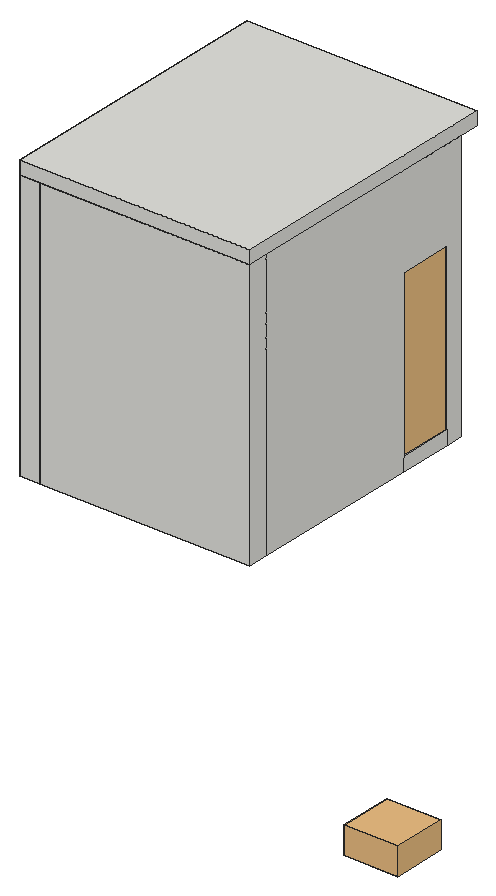
# SketchUp Ruby script. Lengths in inches.
U = 1.inch
M = Sketchup.active_model
def pt(a) = Geom::Point3d.new(a.map { |v| v * U })
def face(e, loops, mat)
  f = e.add_face(loops[0].map { |a| pt(a) })
  loops[1..].each { |l| e.add_face(l.map { |a| pt(a) }).erase! }
  f.material = f.back_material = mat if mat
  f
end
# faces: each face lists its corners as indices into pts; further lists are holes
def faces(e, pts, list, mat = nil) = list.each { |f| face(e, (f[0].is_a?(Array) ? f : [f]).map { |l| l.map { |i| pts[i] } }, mat) }
# xy, xz, yz: faces in a plane at the given z, y or x. An outline is a flat list of corners, or four numbers for a rectangle; further outlines are holes
def ring(l) = l.size == 4 ? [[l[0], l[1]], [l[2], l[1]], [l[2], l[3]], [l[0], l[3]]] : l.each_slice(2).to_a
def flat(e, list, mat, &to3) = list.each { |f| face(e, (f[0].is_a?(Array) ? f : [f]).map { |l| ring(l).map { |u, v| to3.(u, v) } }, mat) }
def xy(e, z, list, mat = nil) = flat(e, list, mat) { |x, y| [x, y, z] }
def xz(e, y, list, mat = nil) = flat(e, list, mat) { |x, z| [x, y, z] }
def yz(e, x, list, mat = nil) = flat(e, list, mat) { |y, z| [x, y, z] }
def lines(e, pts, list) = list.each { |a, b| e.add_line(pt(pts[a]), pt(pts[b])) }
# prism: a flat outline (further loops are holes) pulled along v
def prism(e, loops, v, mat = nil)
  f = face(e, loops, mat); d = Geom::Vector3d.new(v.map { |x| x * U })
  f.pushpull(f.normal.samedirection?(d) ? d.length : -d.length)
end
def box(e, o, s, mat = nil) = prism(e, [[o, [o[0] + s[0], o[1], o[2]], [o[0] + s[0], o[1] + s[1], o[2]], [o[0], o[1] + s[1], o[2]]]], [0, 0, s[2]], mat)
def at(x, y, z, deg = 0) = Geom::Transformation.translation(pt([x, y, z])) * Geom::Transformation.rotation(ORIGIN, Z_AXIS, deg.degrees)
def axes(o, x, y, z) = Geom::Transformation.new([*x, 0, *y, 0, *z, 0, *pt(o).to_a, 1])
def part(name) = M.definitions.add(name)
# library, detail: a bought-in or finely detailed component or shape, given as its bounding box
def library(name, o, s) = part(name).tap { |d| box(d.entities, o, s) }
def detail(e, o, s) = box(e.add_group.entities, o, s)
def put(e, d, t, mat = nil) = e.add_instance(d, t).tap { |i| i.material = mat if mat }
def group(e, t, mat = nil) = e.add_group.tap { |g| g.transformation = t; g.material = mat if mat }.entities
root = M.entities
M.materials.add("ATBTOALHA").color = [214, 222, 215]
M.materials.add("Aluminum_Bumpy_5cm\#2").color = [83, 85, 85]
M.materials.add("Material \#2145965240").color = [200, 201, 192]
M.materials.add("Material \#2145965245").color = [91, 110, 63]
M.materials.add("Material \#33").color = [95, 70, 46]
M.materials.add("Material \#34").color = [97, 116, 28]
M.materials.add("R842VGX RIFLESSO CARPET 200X300 SMOKE").color = [156, 152, 152]
M.materials.add("TEXTURE").color = [202, 201, 217]
M.materials.add("TEXTURE\#1").color = [208, 182, 215]
M.materials.add("TEXTURE\#2").color = [208, 164, 194]
M.materials.add("TILE").color = [214, 172, 168]
M.materials.add("Wood_232").color = [187, 187, 187]
M.materials.add("[Color M07]").color = [58, 58, 58]
M.materials.add("[Mirror 01]").color = [185, 185, 185]
M.materials.add("[Stone Vein Gray]").color = [166, 165, 165]
M.materials.add("glass").color = [129, 129, 129]
M.materials["glass"].alpha = 0.1
M.materials.add("mirror\#1").color = [129, 129, 129]
M.materials.add("staklo kabina1").color = [198, 204, 204]
M.materials["staklo kabina1"].alpha = 0.1
c1 = library("Cabinet pull",[-0.17,-0.54,-0.33],[4.53,0.54,0.66])
c2 = library("K-16141 Revival® toilet tissue holder",[-4.0625,-2.67,-4.49],[8.125,5.34,8.98])
c3 = part("Group\#48")
xy(c3.entities,0,[[0,0,0.39,22.64]])
xy(c3.entities,78.54,[[0,0,0.39,22.64]])
xz(c3.entities,0,[[0,0,0.39,78.54]])
xz(c3.entities,22.64,[[0,0,0.39,78.54]])
yz(c3.entities,0,[[0,0,22.64,78.54]])
yz(c3.entities,0.39,[[0,0,22.64,78.54]],"glass")
c4 = part("Shower screen")
put(c4.entities,c3,axes([1.18,7.5625,0.2],[1,0,0],[0,0.83439,0],[0,0,1]),"staklo kabina1")
g1 = group(c4.entities,at(1.77,49.04,22.15),"Aluminum_Bumpy_5cm\#2")
prism(g1,[[[-0.1875,2.58,48.72],[-0.1875,2.58,47.74],[-0.1875,1.44,47.74],[-0.1875,1.44,46.26],[-0.1875,2.58,46.26],[-0.1875,2.58,45.28],[-0.1875,0,45.28],[-0.1875,0,48.72]]],[0.1875,0,0],"Aluminum_Bumpy_5cm\#2")
prism(g1,[[[-0.6,2.58,45.28],[-0.6,2.58,46.26],[-0.6,1.44,46.26],[-0.6,1.44,47.74],[-0.6,2.58,47.74],[-0.6,2.58,48.72],[-0.6,0,48.72],[-0.6,0,45.28]]],[-0.1875,0,0],"Aluminum_Bumpy_5cm\#2")
prism(g1,[[[0,2.58,-14.15],[0,2.58,-13.17],[0,1.44,-13.17],[0,1.44,-11.69],[0,2.58,-11.69],[0,2.58,-10.71],[0,0,-10.71],[0,0,-14.15]]],[-0.1875,0,0],"Aluminum_Bumpy_5cm\#2")
prism(g1,[[[-0.6,2.58,-14.15],[-0.6,2.58,-13.17],[-0.6,1.44,-13.17],[-0.6,1.44,-11.69],[-0.6,2.58,-11.69],[-0.6,2.58,-10.71],[-0.6,0,-10.71],[-0.6,0,-14.15]]],[-0.1875,0,0],"Aluminum_Bumpy_5cm\#2")
xy(g1,-22.15,[[-0.79,2.64,-0.79,5.16,-0.6,5.16,-0.6,2.86,-0.1875,2.86,-0.1875,5.16,0,5.16,0,2.64]],"Aluminum_Bumpy_5cm\#2")
xy(g1,-13.12,[[-0.75,1.49,-0.04,2.64]],"Aluminum_Bumpy_5cm\#2")
xy(g1,-11.74,[[-0.75,1.49,-0.04,2.64]],"Aluminum_Bumpy_5cm\#2")
xy(g1,46.31,[[-0.75,1.49,-0.04,2.64]],"Aluminum_Bumpy_5cm\#2")
xy(g1,47.6875,[[-0.75,1.49,-0.04,2.64]],"Aluminum_Bumpy_5cm\#2")
xy(g1,56.59,[[-0.79,2.64,0,2.64,0,5.16,-0.1875,5.16,-0.1875,2.86,-0.6,2.86,-0.6,5.16,-0.79,5.16]],"Aluminum_Bumpy_5cm\#2")
xz(g1,1.49,[[-0.75,-13.12,-0.04,-11.74],[-0.75,46.31,-0.04,47.6875]],"Aluminum_Bumpy_5cm\#2")
xz(g1,2.64,[[-0.79,-22.15,0,-22.15,0,-13.12,-0.75,-13.12,-0.75,-11.74,0,-11.74,0,-10.71,-0.79,-10.71],[-0.75,-13.12,-0.04,-11.74],[-0.04,-13.12,0,-11.74],[-0.79,-10.71,0,-10.71,0,46.31,-0.75,46.31,-0.75,47.6875,0,47.6875,0,56.59,-0.79,56.59],[-0.75,46.31,-0.04,47.6875],
  [-0.04,46.31,0,47.6875]],"Aluminum_Bumpy_5cm\#2")
xz(g1,2.86,[[-0.6,-22.15,-0.1875,-10.71],[-0.6,-10.71,-0.1875,56.59]],"Aluminum_Bumpy_5cm\#2")
xz(g1,5.16,[[-0.79,-22.15,-0.6,-10.71],[-0.1875,-22.15,0,-10.71],[-0.79,-10.71,-0.6,56.59],[-0.1875,-10.71,0,56.59]],"Aluminum_Bumpy_5cm\#2")
yz(g1,-0.79,[[2.64,-22.15,5.16,56.59]],"Aluminum_Bumpy_5cm\#2")
yz(g1,-0.75,[[1.49,-13.12,2.64,-11.74],[1.49,46.31,2.64,47.6875]],"Aluminum_Bumpy_5cm\#2")
yz(g1,-0.6,[[2.86,-22.15,5.16,-10.71],[2.86,-10.71,5.16,56.59]],"Aluminum_Bumpy_5cm\#2")
yz(g1,-0.1875,[[2.86,-22.15,5.16,-10.71],[2.86,-10.71,5.16,56.59]],"Aluminum_Bumpy_5cm\#2")
yz(g1,-0.04,[[1.49,-13.12,2.64,-11.74],[1.49,46.31,2.64,47.6875]],"Aluminum_Bumpy_5cm\#2")
yz(g1,0,[[2.64,-22.15,5.16,-10.71],[2.64,-10.71,5.16,56.59]],"Aluminum_Bumpy_5cm\#2")
put(c4.entities,c3,axes([1.18,32.8,0.2],[1,0,0],[0,0.83439,0],[0,0,1]),"staklo kabina1")
c5 = library("Soap Dispenser 22-65",[-1.36,-1.375,0],[2.72,2.74,6.26])
c6 = library("Soap Dispenser 22-61",[-1.33,-1.57,0],[2.66,2.9,5.94])
c7 = library("Bath Accessories 003",[-1.27,-0.78,0],[2.49,1.57,5.35])
c8 = part("taoru")
prism(c8.entities,[[[8.78,1.24,0],[8.78,9.36,0],[8.78,9.36,1.08],[8.78,9.87,1.08],[8.78,9.87,2.17],[8.78,7.84,2.48],[8.78,1.24,2.48],[8.78,0.36,2.12],[8.78,0,1.24],[8.78,0.36,0.36]]],[-8.78,0,0],"ATBTOALHA")
p = [[0,9.36,1.08],[0,1.09,1.08],[8.78,9.36,1.08],[8.78,1.16,1.08]]
lines(c8.entities,p,[[0,1],[2,3]])
c9 = library("skp31A6",[-6.04,-1.48,32.125],[7.16,7.43,5.2])
c10 = library("skp31A6\#1",[-6.04,-1.48,32.125],[7.16,7.43,5.2])
c11 = library("PLANT-201_Defintion",[-475.32,-472.83,-28.125],[950.75,945.66,1000])
c12 = part("Group6\#1")
put(c12.entities,c11,axes([-44342.57,-2801.69,26416.98],[1.62038,0,0],[0,1.62038,0],[0,0,1.62038]),"Material \#2145965240")
c13 = library("PLANT-203_Defintion2",[-533.5,-493.98,-28.55],[984.83,1000,699.26])
c14 = library("PLANT-203_Defintion",[-526.625,-500.29,-11.57],[977.76,1000,668.71])
c15 = part("Group8\#3")
put(c15.entities,c13,axes([-44281.1875,-2905.46,27781.71],[0.88641,-1.61253,0],[1.61253,0.88641,0],[0,0,1.8685]),"Material \#34")
put(c15.entities,c14,axes([-44281.1875,-2905.46,27781.71],[0.9729,-1.76986,0],[1.76986,0.9729,0],[0,0,2.0508]),"Material \#2145965245")
c16 = part("Group7\#1")
put(c16.entities,c15,at(0,0,0))
c17 = library("PLANT-202_Defintion",[-500,-500,-15.45],[999.99,1000,259.15])
c18 = part("Group9\#1")
put(c18.entities,c17,axes([-44334.28,-2800.6875,27750.31],[0,1.46952,0],[-1.46952,0,0],[0,0,1.13496]),"Material \#33")
c19 = part("Group5\#1")
put(c19.entities,c12,at(0,0,0))
put(c19.entities,c16,at(0,0,0))
put(c19.entities,c18,at(0,0,0))
c20 = part("PLANTING")
g2 = group(c20.entities,at(4454.16,289.51,-2634.93))
put(g2,c19,axes([0,0,0],[0.1,0,0],[0,0.1,0],[0,0,0.1]))
c21 = part("DDR842RVS01100X")
xy(c21.entities,0,[[-70.87,0,47.24,78.74]])
xy(c21.entities,0.39,[[-70.87,0,47.24,78.74]],"R842VGX RIFLESSO CARPET 200X300 SMOKE")
xz(c21.entities,0,[[-70.87,0,47.24,0.39]])
xz(c21.entities,78.74,[[-70.87,0,47.24,0.39]])
yz(c21.entities,-70.87,[[0,0,78.74,0.39]])
yz(c21.entities,47.24,[[0,0,78.74,0.39]])
c22 = library("OralB_Pro6000_Toothbrush",[-0.05,-0.01,-0.01],[13.51,3.44,10.23])
c23 = library("Dome Light",[-12,-12,0],[24,24,12])
c24 = library("Group\#6",[0,0,-9.3125],[12,18,14.04])
c25 = library("Group\#15",[0,0,0],[24.35,24.35,4.73])
c26 = library("Group\#73",[0.12,0.01,0],[2.52,3.27,6.75])
c27 = library("组\#30",[-0.73,0,0],[12.16,12.33,14.02])
c28 = library("Group\#61",[0,0,0],[8.67,43.49,8.21])
c29 = library("Group\#78",[0,0,0],[3.37,3.05,7.71])
c30 = library("Group\#11",[0,0,0],[25.8,16.01,34.24])
c31 = library("Group\#10",[0,0,0],[12.05,13.22,9.68])
c32 = library("Group\#151",[0,0,0],[10.375,9.6,13.04])
c33 = library("Group\#57",[0,0,0],[15.12,15.37,8.71])
c34 = library("Group\#98",[0,0,0],[34.65,5.6,83.07])
c35 = library("Rectangle Light",[-3.49,-3.49,-3.49],[6.98,6.98,3.49])
c36 = library("Recessed downlight",[0,0,-6],[8.36,8.36,6.5])
xy(root,73.16,[[16.958,15.874,16.866,15.891,16.916,15.909],[16.958,15.874,16.916,15.909,16.969,15.928],[16.958,15.874,16.969,15.928,17.023,15.948],[16.861,15.889,16.862,15.891,16.859,15.892],[16.861,15.889,16.866,15.891,16.862,15.891],
  [16.862,15.891,16.879,15.939,16.789,16.014,16.859,15.892],[16.862,15.891,16.879,15.939,16.916,15.909,16.866,15.891],[16.859,15.892,16.811,15.901,16.758,16.039,16.789,16.014],[16.916,15.909,16.879,15.939,16.939,16.102,16.959,16.11,16.991,16.032,16.969,15.928],[16.969,15.928,16.991,16.032,17.025,15.951,17.023,15.948],
  [16.879,15.939,16.789,16.014,16.773,16.041,16.795,16.052,16.939,16.102],[17.023,15.948,17.026,15.949,17.025,15.951],[17.025,15.951,16.991,16.032,17.012,16.128,17.056,15.986],[16.789,16.014,16.758,16.039,16.795,16.052,16.773,16.041],[16.991,16.032,16.959,16.11,17.012,16.128],
  [16.758,16.039,16.856,16.157,17.012,16.128,16.959,16.11,16.95,16.133,16.795,16.052],[16.795,16.052,16.939,16.102,16.95,16.133],[16.939,16.102,16.959,16.11,16.95,16.133]])
xy(root,73.555,[[17.034,15.767,16.759,15.779,16.949,15.876,16.967,15.885,17.187,15.997],[16.759,15.779,16.626,16.02,16.763,16.258,16.761,16.044,16.758,16.039,16.761,16.03],[16.759,15.779,16.761,16.03,16.811,15.901,16.949,15.876],[16.958,15.874,16.967,15.885,16.949,15.876],[16.949,15.876,16.811,15.901,17.056,15.986,16.967,15.885],
  [16.967,15.885,17.056,15.986,17.021,16.099,17.187,15.997],[16.811,15.901,16.761,16.03,16.761,16.044,16.856,16.157],[16.811,15.901,16.856,16.157,17.056,15.986],[17.056,15.986,17.021,16.099,16.958,16.138,16.856,16.157],[17.187,15.997,17.021,16.099,17.012,16.128,16.958,16.138,16.763,16.258,17.065,16.247],
  [16.761,16.03,16.758,16.039,16.761,16.044],[16.761,16.044,16.763,16.258,16.958,16.138,16.856,16.157],[17.021,16.099,16.958,16.138,17.012,16.128]])
xy(root,75.002,[[17.034,15.767,17.187,15.997,16.759,15.779],[16.759,15.779,16.763,16.258,16.626,16.02],[16.759,15.779,17.187,15.997,16.763,16.258],[17.187,15.997,17.065,16.247,16.763,16.258]])
p = [[16.888,15.889,71.969],[16.8,16.041,71.965],[16.942,16.041,70.178],[17.053,15.949,71.976],[17.03,15.889,70.188],[17.118,16.133,70.198],
  [17.194,15.949,70.207],[16.976,16.133,71.973],[16.861,15.889,73.16],[16.859,15.892,73.16],[16.789,16.014,73.16],[16.773,16.041,73.16],
  [17.026,15.949,73.16],[17.023,15.948,73.16],[16.969,15.928,73.16],[16.916,15.909,73.16],[16.866,15.891,73.16],[16.95,16.133,73.16],
  [16.959,16.11,73.16],[16.991,16.032,73.16],[17.025,15.951,73.16],[16.795,16.052,73.16],[16.758,16.039,73.16],[16.811,15.901,73.16],
  [16.811,15.901,73.555],[16.761,16.03,73.555],[16.758,16.039,73.555],[16.862,15.891,73.16],[16.958,15.874,73.16],[16.958,15.874,73.555],
  [16.949,15.876,73.555],[17.056,15.986,73.16],[17.056,15.986,73.555],[16.967,15.885,73.555],[16.856,16.157,73.16],[16.761,16.044,73.555],
  [16.856,16.157,73.555],[17.012,16.128,73.16],[17.012,16.128,73.555],[17.021,16.099,73.555],[16.958,16.138,73.555],[16.759,15.779,75.002],
  [16.626,16.02,75.002],[16.626,16.02,73.555],[16.759,15.779,73.555],[17.034,15.767,75.002],[17.034,15.767,73.555],[17.187,15.997,73.555],
  [17.187,15.997,75.002],[16.763,16.258,75.002],[16.763,16.258,73.555],[17.065,16.247,73.555],[17.065,16.247,75.002],[34.783,55.903,21.959],
  [35.783,55.903,21.959],[35.783,56.903,21.959]]
faces(root,p,[[0,1,2],[3,0,4],[2,4,0],[4,2,5],[4,6,3],[6,5,7],[7,3,6],[5,6,4],
  [5,2,1],[1,7,5],[1,0,8],[8,9,10,11,1],[0,3,12],[12,13,14,15,16,8,0],[3,7,17],[17,18,19,20,12,3],
  [7,1,11],[11,21,17,7],[22,23,24],[24,25,26,22],[23,9,27,16,28,29],[29,30,24,23],[28,13,20,31,32],[32,33,29,28],
  [34,22,26],[26,35,36,34],[31,37,38],[38,39,32,31],[37,34,36],[36,40,38,37],[41,42,43],[43,44,41],
  [45,41,44],[44,46,45],[45,46,47],[47,48,45],[49,50,43],[43,42,49],[48,47,51],[51,52,48],
  [49,52,51],[51,50,49]])
lines(root,p,[[53,54],[54,55],[55,53]])
detail(root,[15.45,14.57,69.71],[2.89,2.91,5.17])
put(root,c1,at(39,77.95,40.47,90))
put(root,c1,at(39,91.26,40.47,90))
put(root,c1,at(39,98.33,40.47,90))
put(root,c2,axes([11.06,64.77,29.94],[0,0.77,0],[-0.77,0,0],[0,0,0.77]))
put(root,c4,axes([105.26,37.22,6],[0,1,0],[-1.77611,0,0],[0,0,1.3716]),"Wood_232")
put(root,c5,at(20.92,72.01,42))
put(root,c6,at(12.85,71.6,42))
put(root,c7,at(7.43,72.24,52))
put(root,c8,axes([11.96,50.1,66.72],[0,1.2402,0],[0.9153,0,0],[0,0,0.75]),"Wood_232")
put(root,c8,axes([11.96,50.1,64.86],[0,1.2402,0],[0.9153,0,0],[0,0,0.75]),"Wood_232")
put(root,c8,axes([11.96,50.1,70.2],[0,1.2402,0],[0.9153,0,0],[0,0,0.75]),"Wood_232")
put(root,c8,axes([11.96,50.1,68.34],[0,1.2402,0],[0.9153,0,0],[0,0,0.75]),"Wood_232")
put(root,c9,at(31.51,74.64,-19.125))
put(root,c10,axes([26.21,73.71,-18.48],[0,-1.04733,0],[1.17963,0,0],[0,0,1.10246]))
put(root,c20,axes([16.22,55.42,74.79],[0.03016,0,0],[0,0.03016,0],[0,0,0.03016]))
put(root,c21,axes([69.28,43.67,6],[0.424,0,0],[0,0.424,0],[0,0,0.424]))
put(root,c22,axes([5.01,110.27,52.01],[0,-1,0],[0.87171,0,0],[0,0,1]))
put(root,c23,at(267.22,-127.24,0))
g3 = group(root,at(9,9,0))
xy(g3,0,[[0,0,0,108,84,108,84,100.51,93,100.51,93,76.51,84,76.51,84,0]])
xy(g3,6,[[0,0,84,0,84,76.51,93,76.51,93,100.51,84,100.51,84,108,0,108]],"[Stone Vein Gray]")
xz(g3,0,[[0,0,84,6]])
xz(g3,76.51,[[84,0,93,6]])
xz(g3,100.51,[[84,0,93,6]])
xz(g3,108,[[0,0,84,6]])
yz(g3,0,[[0,0,108,6]])
yz(g3,84,[[0,0,76.51,6],[100.51,0,108,6]])
yz(g3,93,[[76.51,0,100.51,6]])
g4 = group(root,at(9,69,12),"[Color M07]")
xy(g4,0,[[0,0,30,42]])
xy(g4,1,[[0,1,30,41]],"[Color M07]")
xy(g4,13.8125,[[0,1,30,41]])
xy(g4,14,[[29,13.92,30,14.08],[29,27.92,30,28.08]])
xy(g4,29,[[0,0,30,0,30,13.92,29,13.92,29,14.08,30,14.08,30,27.92,29,27.92,29,28.08,30,28.08,30,42,0,42]])
xz(g4,0,[[0,0,30,29]],"TEXTURE\#2")
xz(g4,1,[[0,1,30,13.8125]],"[Color M07]")
xz(g4,13.92,[[29,14,30,29]])
xz(g4,14.08,[[29,14,30,29]])
xz(g4,27.92,[[29,14,30,29]])
xz(g4,28.08,[[29,14,30,29]])
xz(g4,41,[[0,1,30,13.8125]],"[Color M07]")
xz(g4,42,[[0,0,30,29]],"[Color M07]")
yz(g4,0,[[[0,0,42,29],[1,1,41,13.8125]]])
yz(g4,29,[[13.92,14,14.08,29],[27.92,14,28.08,29]])
yz(g4,30,[[[0,0,42,14],[1,1,41,13.8125]],[0,14,13.92,29],[14.08,14,27.92,29],[28.08,14,42,29]],"[Color M07]")
g5 = group(root,at(9,68.53,41),"TILE")
box(g5,[0,0,0],[30.47,42.94,1],"TILE")
put(root,c24,at(9,44.58,74.17))
g6 = group(root,at(9,44.58,64.17))
box(g6,[0,0,0],[12,18,0.6875])
g7 = group(root,at(0,0,0))
xy(g7,0,[[9,0,102,9]])
xy(g7,58.68,[[47.62,6,58.62,9]])
xy(g7,66.8,[[47.62,6,58.62,9]])
xy(g7,120,[[9,0,102,9]])
xz(g7,0,[[9,0,102,120]])
xz(g7,6,[[47.62,58.68,58.62,66.8]])
xz(g7,9,[[[9,0,102,120],[47.62,58.68,58.62,66.8]]],"TEXTURE\#1")
yz(g7,9,[[0,0,9,120]])
yz(g7,47.62,[[6,58.68,9,66.8]])
yz(g7,58.62,[[6,58.68,9,66.8]])
yz(g7,102,[[0,0,9,120]])
g8 = group(root,at(0,9,0))
g9 = group(g8,at(0,-9,0))
xy(g9,0,[[0,0,9,117]])
xy(g9,42,[[8,69,9,111]])
xy(g9,52,[[5,69,8,111]])
xy(g9,56,[[4,69,5,111]])
xy(g9,102,[[4,69,5,111]])
xy(g9,120,[[0,0,9,0,9,69,5,69,5,111,9,111,9,117,0,117]])
xz(g9,0,[[0,0,9,120]])
xz(g9,69,[[8,42,8,52,5,52,5,56,4,56,4,102,5,102,5,120,9,120,9,42]],"[Color M07]")
xz(g9,111,[[8,42,9,42,9,120,5,120,5,102,4,102,4,56,5,56,5,52,8,52]],"TEXTURE")
xz(g9,117,[[0,0,9,120]])
yz(g9,0,[[0,0,117,120]])
yz(g9,4,[[70,56,110,100]],"[Mirror 01]")
yz(g9,4,[[69,56,70,100],[110,56,111,100],[69,100,111,102]],"mirror\#1")
yz(g9,5,[[69,102,111,120]],"TEXTURE\#2")
yz(g9,5,[[69,52,111,56]],"mirror\#1")
yz(g9,8,[[69,42,111,52]],"TEXTURE\#2")
yz(g9,9,[[0,0,117,0,117,120,111,120,111,42,69,42,69,120,0,120]],"[Color M07]")
put(root,c25,at(3.4,1.56,68.64))
put(root,c26,axes([13.15,19.11,69.33],[0.85,0,0],[0,0.85,0],[0,0,1]))
put(root,c27,axes([12.93,10.0625,69.33],[0,0.46332,0],[0.46332,0,0],[0,0,0.46332]))
put(root,c28,axes([70.9375,9,44.47],[-1,0,0],[0,0,1.04],[0,1,0]),"Wood_232")
g10 = group(root,at(93,38.2,6),"Aluminum_Bumpy_5cm\#2")
xy(g10,0,[[-34.64,0,0,0.79]])
xy(g10,0.27,[[-34.64,0.2,-1.16,0.59]])
xy(g10,1.08,[[-34.64,0,-1.16,0.2],[-34.64,0.59,-1.16,0.79]])
xy(g10,108,[[-1.16,0,0,0.79]])
xz(g10,0,[[-34.64,0,0,0,0,108,-1.16,108,-1.16,1.08,-34.64,1.08]])
xz(g10,0.2,[[-34.64,0.27,-1.16,1.08]])
xz(g10,0.59,[[-34.64,0.27,-1.16,1.08]])
xz(g10,0.79,[[-34.64,0,-1.16,1.08],[-0.875,0.27,-0.875,1.08,-1.16,1.08,-1.16,108,0,108,0,1.08,-0.29,1.08,-0.29,0.27]])
yz(g10,-34.64,[[0,0,0,1.08,0.2,1.08,0.2,0.27,0.59,0.27,0.59,1.08,0.79,1.08,0.79,0]])
yz(g10,-1.16,[[0.2,0.27,0.2,1.08,0,1.08,0,108,0.79,108,0.79,1.08,0.59,1.08,0.59,0.27]])
yz(g10,0,[[0,0,0.79,108]])
put(root,c29,at(15.39,14.5,69.65))
put(root,c30,at(9,44.92,6))
put(root,c31,at(18.61,82.17,13))
g11 = group(root,at(31.7,108.36,13))
xy(g11,0,[[-10.74,-11.76,-10.84,-0.09,0,0,0.1,-11.66]])
xy(g11,0.6,[[-10.38,-11.36,-0.26,-11.28,-0.36,-0.39,-10.47,-0.48]])
xy(g11,9.61,[[[-10.74,-11.76,0.1,-11.66,0,0,-10.84,-0.09],[-10.38,-11.36,-10.47,-0.48,-0.36,-0.39,-0.26,-11.28]]])
p = [[-10.84,-0.09,0],[-10.74,-11.76,0],[-10.74,-11.76,9.61],[-10.84,-0.09,9.61],[0.1,-11.66,0],[0.1,-11.66,9.61],
  [0,0,0],[0,0,9.61],[-10.47,-0.48,9.61],[-10.38,-11.36,9.61],[-10.38,-11.36,0.6],[-10.47,-0.48,0.6],
  [-0.26,-11.28,9.61],[-0.26,-11.28,0.6],[-0.36,-0.39,9.61],[-0.36,-0.39,0.6]]
faces(g11,p,[[0,1,2,3],[1,4,5,2],[4,6,7,5],[6,0,3,7],[8,9,10,11],[9,12,13,10],[12,14,15,13],[14,8,11,15]])
put(root,c32,axes([15.46,52.01,74.86],[0,-0.57691,0],[0.57691,0,0],[0,0,0.61246]))
put(root,c33,at(9,98.91,42,-90))
g12 = group(root,at(93,9,0))
xy(g12,0,[[0,0,9,76.51],[0,100.51,9,108]])
xy(g12,79.2,[[0,76.51,9,100.51]])
xy(g12,120,[[0,0,9,108]])
xz(g12,0,[[0,0,9,120]])
xz(g12,76.51,[[0,0,9,79.2]])
xz(g12,100.51,[[0,0,9,79.2]])
xz(g12,108,[[0,0,9,120]])
yz(g12,0,[[0,0,0,120,108,120,108,0,100.51,0,100.51,79.2,76.51,79.2,76.51,0]],"[Color M07]")
yz(g12,9,[[0,0,76.51,0,76.51,79.2,100.51,79.2,100.51,0,108,0,108,120,0,120]])
put(root,c34,axes([101.16,85.51,6],[0,0.69273,0],[-0.85,0,0],[0,0,0.88119]))
g13 = group(root,at(0,0,110.51))
g14 = group(g13,at(0,0,9.49))
box(g14,[0,0,0],[102,126,6])
g15 = group(g13,at(0,0,0))
put(g15,c35,at(23.94,93,3.49,180))
put(g15,c35,at(51,93,3.49,180))
put(g15,c35,at(78,24,3.49,180))
put(g15,c35,at(51,24,3.49,180))
put(g15,c35,at(78,58.5,3.49,180))
put(g15,c35,at(23.94,24,3.49,180))
put(g15,c35,at(23.94,58.5,3.49,180))
put(g15,c35,at(78,93,3.49,180))
g16 = group(g15,at(0,0,3.49))
box(g16,[9,9,0],[84,108,6])
put(g16,c36,axes([82.18,88.82,0],[-1,0,0],[0,1,0],[0,0,-1]))
put(g16,c36,axes([55.18,88.82,0],[-1,0,0],[0,1,0],[0,0,-1]))
put(g16,c36,axes([28.18,88.82,0],[-1,0,0],[0,1,0],[0,0,-1]))
put(g16,c36,axes([28.18,54.32,0],[-1,0,0],[0,1,0],[0,0,-1]))
put(g16,c36,axes([82.18,54.32,0],[-1,0,0],[0,1,0],[0,0,-1]))
put(g16,c36,axes([28.18,19.82,0],[-1,0,0],[0,1,0],[0,0,-1]))
put(g16,c36,axes([55.18,19.82,0],[-1,0,0],[0,1,0],[0,0,-1]))
put(g16,c36,axes([82.18,19.82,0],[-1,0,0],[0,1,0],[0,0,-1]))
